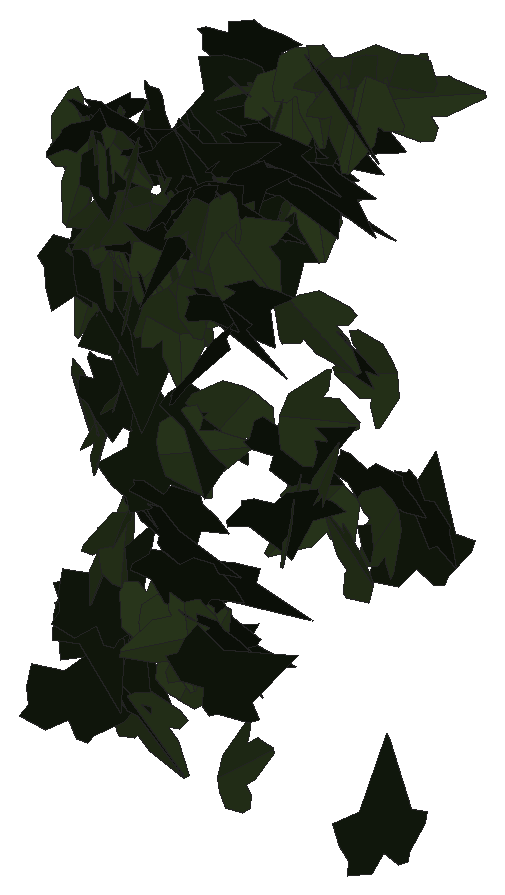
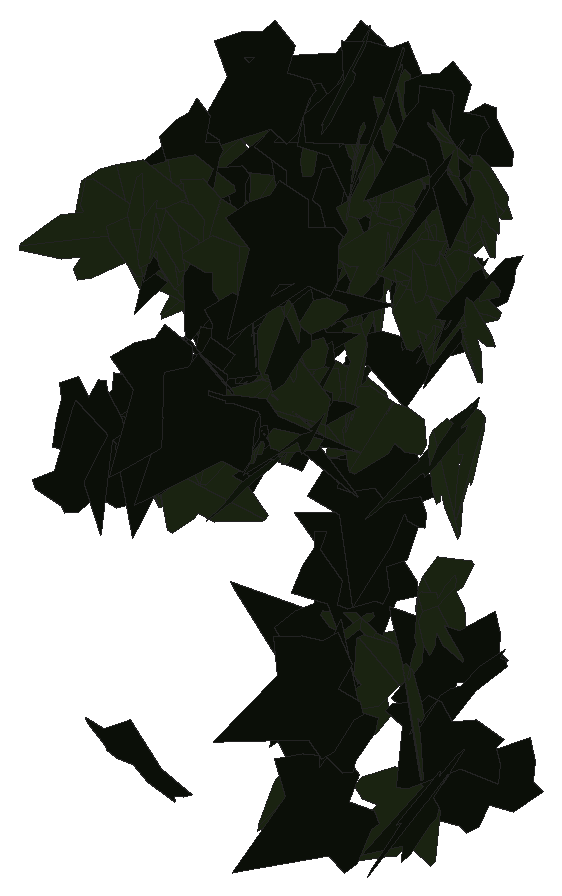
# SketchUp Ruby script. Lengths in inches.
U = 1.inch
M = Sketchup.active_model
def pt(a) = Geom::Point3d.new(a.map { |v| v * U })
def face(e, loops, mat)
  f = e.add_face(loops[0].map { |a| pt(a) })
  loops[1..].each { |l| e.add_face(l.map { |a| pt(a) }).erase! }
  f.material = f.back_material = mat if mat
  f
end
# faces: each face lists its corners as indices into pts; further lists are holes
def faces(e, pts, list, mat = nil) = list.each { |f| face(e, (f[0].is_a?(Array) ? f : [f]).map { |l| l.map { |i| pts[i] } }, mat) }
# xy, xz, yz: faces in a plane at the given z, y or x. An outline is a flat list of corners, or four numbers for a rectangle; further outlines are holes
def ring(l) = l.size == 4 ? [[l[0], l[1]], [l[2], l[1]], [l[2], l[3]], [l[0], l[3]]] : l.each_slice(2).to_a
def flat(e, list, mat, &to3) = list.each { |f| face(e, (f[0].is_a?(Array) ? f : [f]).map { |l| ring(l).map { |u, v| to3.(u, v) } }, mat) }
def xy(e, z, list, mat = nil) = flat(e, list, mat) { |x, y| [x, y, z] }
def xz(e, y, list, mat = nil) = flat(e, list, mat) { |x, z| [x, y, z] }
def yz(e, x, list, mat = nil) = flat(e, list, mat) { |y, z| [x, y, z] }
def lines(e, pts, list) = list.each { |a, b| e.add_line(pt(pts[a]), pt(pts[b])) }
# prism: a flat outline (further loops are holes) pulled along v
def prism(e, loops, v, mat = nil)
  f = face(e, loops, mat); d = Geom::Vector3d.new(v.map { |x| x * U })
  f.pushpull(f.normal.samedirection?(d) ? d.length : -d.length)
end
def box(e, o, s, mat = nil) = prism(e, [[o, [o[0] + s[0], o[1], o[2]], [o[0] + s[0], o[1] + s[1], o[2]], [o[0], o[1] + s[1], o[2]]]], [0, 0, s[2]], mat)
def at(x, y, z, deg = 0) = Geom::Transformation.translation(pt([x, y, z])) * Geom::Transformation.rotation(ORIGIN, Z_AXIS, deg.degrees)
def axes(o, x, y, z) = Geom::Transformation.new([*x, 0, *y, 0, *z, 0, *pt(o).to_a, 1])
def part(name) = M.definitions.add(name)
# library, detail: a bought-in or finely detailed component or shape, given as its bounding box
def library(name, o, s) = part(name).tap { |d| box(d.entities, o, s) }
def detail(e, o, s) = box(e.add_group.entities, o, s)
def put(e, d, t, mat = nil) = e.add_instance(d, t).tap { |i| i.material = mat if mat }
def group(e, t, mat = nil) = e.add_group.tap { |g| g.transformation = t; g.material = mat if mat }.entities
root = M.entities
M.materials.add("efeu1").color = [18, 25, 13]
M.materials.add("efeu2").color = [43, 57, 29]
c1 = part("ivyleaf_10")
p = [[0,0.5,-0.03],[-0.0625,2.02,-0.43],[-0.19,2.01,-0.46],[-0.54,1.05,-0.29],[-0.52,0.625,-0.18],[-0.83,0.76,-0.28],
  [-1.16,0.64,-0.33],[-1.15,0.33,-0.24],[-0.77,-0.39,0.02],[-0.3,-0.51,0.16],[0.04,-0.48,0.23],[-0.02,2.01,-0.4375],
  [-0.06,2.01,-0.43],[0.04,-0.49,0.23],[0.67,-0.49,0.14],[1.38,0.36,-0.2],[1.375,0.51,-0.24],[0.81,0.65,-0.19],
  [0.62,0.59,-0.15],[0.6,1.09,-0.28],[0.5,1.23,-0.31]]
faces(c1.entities,p,[[0,1,2,3,4,5,6,7,8,9,10],[11,12,0,13,14,15,16,17,18,19,20]],"efeu2")
c2 = part("ivyleaf_9")
p = [[1.54,2.16,1.25],[1.36,2.04,1.19],[-0.21,0.99,0.68],[-0.71,1.11,0.82],[-0.85,0.86,0.67],[-0.8,0.17,0.21],
  [-0.9,-0.01,0.1],[-0.67,-0.16,-0.02],[-0.08,-0.08,-0.05],[-0.03,-0.6,-0.4],[0.65,-0.88,-0.66],[0.83,-0.6,-0.49],
  [1.29,-0.42,-0.43],[1.8125,-0.07,-0.26],[1.21,0.44,0.15]]
faces(c2.entities,p,[[0,1,2,3,4,5,6,7,8,9,10,11,12,13,14]],"efeu1")
put(root,c1,axes([31.71,224.67,222.89],[0.24718,-0.43455,-0.00798],[-0.00248,0.00777,-0.49993],[0.43462,0.24719,0.00168]))
put(root,c1,axes([32.43,224.52,218.62],[0.11399,0.02563,-0.48616],[0.48525,0.0343,0.11558],[0.03927,-0.49816,-0.01706]))
put(root,c1,axes([30.8,224.67,222.25],[0.47412,-0.15396,-0.03882],[-0.03543,0.01656,-0.49847],[0.15478,0.47542,0.00479]))
put(root,c2,axes([30.73,224.47,214.24],[-0.19479,-0.11689,0.44541],[0.44193,0.08849,0.21649],[-0.12944,0.47802,0.06884]))
put(root,c2,axes([30.93,224.76,220.62],[0.25939,-0.42519,0.04395],[0.01945,-0.03961,-0.49805],[0.42701,0.26008,-0.00401]))
put(root,c1,axes([32.38,224.51,220.8125],[-0.24257,-0.36838,-0.23549],[0.15079,0.1823,-0.44049],[0.41039,-0.28472,0.02265]))
put(root,c1,axes([32.86,224.7,222.33],[-0.46609,0.17503,0.04604],[-0.1086,-0.16874,-0.45797],[-0.14478,-0.43691,0.19531]))
put(root,c2,axes([33.23,224.4,221.14],[0.34783,0.35872,-0.01827],[-0.01238,-0.01345,-0.49967],[-0.35897,0.34805,-0.00048]))
put(root,c1,axes([34.41,224.58,221.26],[-0.40164,-0.04492,-0.29439],[0.29289,0.02981,-0.40414],[0.05386,-0.49709,0.00237]))
put(root,c1,axes([31.16,224.86,216.9],[0.08879,-0.45136,0.19593],[0.05541,-0.18866,-0.45971],[0.48892,0.10335,0.01652]))
put(root,c1,axes([31.9,224.62,221.79],[-0.2401,-0.42699,-0.10015],[0.05178,0.08578,-0.48986],[0.43551,-0.2456,0.00303]))
put(root,c1,axes([32.3,225.01,215.7],[-0.07669,0.06285,0.49007],[-0.12924,-0.48122,0.04149],[0.47688,-0.12031,0.09005]))
put(root,c1,axes([32.32,224.65,220.55],[0.21033,0.45351,-0.00953],[-0.01614,-0.00301,-0.49973],[-0.45332,0.21053,0.01337]))
put(root,c1,axes([31.14,224.75,218.67],[0.1504,-0.47684,-0.00062],[-0.00017,0.00059,-0.5],[0.47684,0.1504,0.00001]))
put(root,c1,axes([30.92,224.74,220.64],[0.45441,-0.20734,-0.02286],[-0.02024,0.0107,-0.49948],[0.20761,0.45486,0.00133]))
put(root,c2,axes([32.42,224.47,222.59],[0.12712,-0.00695,0.48352],[0.4742,0.09971,-0.12323],[-0.09472,0.48991,0.03194]))
put(root,c2,axes([32.79,224.64,215.32],[0.01174,-0.00596,0.49983],[0.47668,-0.15037,-0.01299],[0.15048,0.47681,0.00215]))
put(root,c1,axes([30.81,224.58,218.9],[-0.35201,0.35299,0.03855],[-0.02671,0.0278,-0.49851],[-0.35408,-0.35302,-0.00072]))
put(root,c2,axes([32.2,224.53,217.86],[0.39157,0.21964,-0.22007],[-0.18354,-0.12237,-0.44871],[-0.25097,0.43218,-0.01521]))
put(root,c2,axes([30.82,224.8,215.8],[0.1121,-0.47584,-0.1049],[-0.01642,0.10389,-0.48881],[0.48699,0.11304,0.00766]))
put(root,c2,axes([32.41,224.93,221.93],[-0.1708,0.17047,-0.43792],[0.25145,-0.36047,-0.23839],[-0.39699,-0.30166,0.03741]))
put(root,c1,axes([32.75,224.72,222.21],[-0.05325,-0.49584,-0.03615],[0.00384,0.03595,-0.49869],[0.49714,-0.05339,-0.00003]))
put(root,c2,axes([32.83,224.33,220.01],[0.04217,0.41055,0.28226],[0.03332,0.28032,-0.41269],[-0.4971,0.05362,-0.00372]))
put(root,c2,axes([30.66,224.6,220.93],[0.1707,-0.32096,-0.34329],[-0.14958,0.30914,-0.3634],[0.44552,0.22677,0.00952]))
put(root,c2,axes([31.93,224.52,221.57],[0.3478,0.33605,-0.12691],[-0.08958,-0.08993,-0.48362],[-0.34786,0.35914,-0.00235]))
put(root,c2,axes([33.98,224.52,218.38],[0.24429,0.41669,-0.12919],[-0.08017,-0.10266,-0.48274],[-0.42883,0.25657,0.01666]))
put(root,c2,axes([32.62,224.55,222.44],[-0.07297,0.49153,-0.05541],[0.01986,-0.05305,-0.49678],[-0.49425,-0.07471,-0.01178]))
put(root,c1,axes([30.62,224.81,222.39],[0.41187,-0.21955,0.17933],[0.19745,-0.00478,-0.45934],[0.20341,0.44919,0.08276]))
put(root,c2,axes([32.49,225.07,218.91],[-0.02125,-0.43785,0.24049],[0.11804,-0.23829,-0.42342],[0.4854,0.03878,0.1135]))
put(root,c1,axes([31.375,224.89,220.61],[0.3098,-0.37447,0.11746],[0.09688,-0.07205,-0.4852],[0.38031,0.32339,0.02792]))
put(root,c2,axes([31.11,224.55,215.7],[-0.17499,-0.12318,0.45189],[0.39781,0.21554,0.21281],[-0.24723,0.43402,0.02257]))
put(root,c2,axes([31.89,224.87,217.04],[0.22565,-0.19208,0.40272],[0.34217,-0.21514,-0.29433],[0.28636,0.40843,0.03435]))
put(root,c2,axes([31.02,224.53,222.85],[0.09351,0.49073,-0.02097],[-0.00451,-0.02048,-0.49956],[-0.49116,0.09362,0.0006]))
put(root,c1,axes([32.7,224.78,222.32],[-0.39165,-0.31006,0.02171],[-0.00919,-0.02335,-0.49937],[0.31069,-0.39155,0.01259]))
put(root,c2,axes([31.94,224.51,222.8125],[0.41511,0.10171,0.2595],[0.23261,0.13003,-0.42306],[-0.15355,0.47196,0.06064]))
put(root,c1,axes([33.36,224.54,221.84],[0.14006,0.39477,0.27303],[0.04804,0.27146,-0.41714],[-0.47757,0.14308,0.03811]))
put(root,c2,axes([31.54,224.94,220.06],[-0.1901,-0.43032,-0.16937],[0.06668,0.15571,-0.47043],[0.45762,-0.20145,-0.00181]))
put(root,c1,axes([34.43,224.41,219.82],[0.01564,0.17434,0.46836],[0.00979,0.46839,-0.17468],[-0.49966,0.01464,0.01124]))
put(root,c2,axes([32.34,224.67,216.85],[0.30708,0.28473,-0.27318],[-0.21335,-0.17139,-0.41846],[-0.33194,0.37357,0.01623]))
put(root,c2,axes([32.45,224.77,223.05],[0.37247,-0.30425,-0.13674],[-0.10726,0.08485,-0.48093],[0.31585,0.3876,-0.00206]))
put(root,c2,axes([33.83,224.74,218.95],[0.4246,0.19249,-0.18074],[0.12785,0.14957,0.45965],[0.23102,-0.43655,0.07779]))
put(root,c2,axes([31.02,224.61,222.96],[0.49825,0.04137,0.00554],[0.00197,0.04302,-0.49814],[-0.04169,0.49643,0.04271]))
put(root,c1,axes([32.24,224.74,222.52],[-0.45202,0.0971,0.1904],[-0.19463,-0.00294,-0.46055],[-0.08832,-0.49047,0.04046]))
put(root,c2,axes([32.6,224.64,222.18],[0.41549,0.06904,0.26944],[0.26911,0.02263,-0.42079],[-0.0703,0.49469,-0.01836]))
put(root,c1,axes([34.58,224.84,219.2],[0.3228,-0.35463,-0.14156],[-0.09819,0.10204,-0.47953],[0.369,0.33738,-0.00376]))
put(root,c1,axes([31.09,224.92,221.34],[-0.00101,-0.49877,0.03504],[0.01326,-0.03506,-0.49859],[0.49982,-0.00008,0.0133]))
put(root,c2,axes([31.64,224.78,220.34],[0.10909,-0.26329,0.41082],[-0.17033,0.37394,0.28488],[-0.45726,-0.20211,-0.00811]))
put(root,c1,axes([30.4375,224.85,222.24],[0.31004,-0.09686,-0.38012],[0.37418,-0.07242,0.32365],[-0.11775,-0.48515,0.02758]))
put(root,c1,axes([31.17,224.92,221.54],[-0.16942,-0.4667,0.05904],[-0.02707,-0.05297,-0.49645],[0.46964,-0.17142,-0.00732]))
put(root,c2,axes([32.69,224.72,220.75],[0.49862,-0.03068,0.02099],[0.02104,0.00017,-0.49956],[0.03064,0.49906,0.00146]))
put(root,c1,axes([31.15,224.92,221.26],[0.35534,-0.08732,0.34075],[0.34693,0.00707,-0.35998],[0.05805,0.49226,0.06562]))
put(root,c1,axes([30.9,224.92,222.41],[0.10755,-0.00432,0.48828],[0.48816,-0.01082,-0.10762],[0.0115,0.49986,0.00189]))
put(root,c2,axes([31.85,224.71,223.16],[0.32303,-0.16332,-0.34493],[-0.30157,0.16771,-0.36184],[0.23389,0.44181,0.00985]))
put(root,c1,axes([32.01,224.89,215.99],[0.4313,0.08029,0.23986],[0.23655,0.03992,-0.43869],[-0.0896,0.49189,-0.00355]))
put(root,c2,axes([32.03,224.8,217.95],[-0.46424,-0.16323,0.08851],[0.08727,0.01854,0.49197],[-0.16389,0.47224,0.01128]))
put(root,c2,axes([30.95,224.75,218.99],[0.39035,-0.21757,-0.22425],[-0.10521,0.24637,-0.42218],[0.2942,0.37678,0.14656]))
put(root,c1,axes([32,224.84,221.4],[0.31732,0.37023,0.11062],[0.04997,0.10262,-0.4868],[-0.38316,0.32,0.02813]))
put(root,c2,axes([33.07,224.68,222.58],[0.19265,0.46047,-0.02912],[-0.00674,-0.02875,-0.49913],[-0.46134,0.19271,-0.00487]))
put(root,c1,axes([31.02,224.92,221.05],[-0.26169,-0.42135,-0.06312],[0.05149,0.04225,-0.49554],[0.42293,-0.26586,0.02128]))
put(root,c1,axes([31.04,225.1875,220.94],[0.10295,0.24488,-0.4236],[-0.30015,-0.31025,-0.2523],[-0.38641,0.30624,0.08312]))
put(root,c1,axes([32.37,224.76,221.79],[-0.17324,0.39852,-0.24732],[-0.09138,0.22992,0.43449],[0.46004,0.19575,-0.00683]))
put(root,c1,axes([33.8,225.15,218.31],[0.30782,-0.32876,0.21718],[0.15483,-0.1525,-0.4503],[0.36232,0.34447,0.00791]))
put(root,c1,axes([31.91,224.9,221.05],[-0.39361,0.28512,0.11738],[-0.13942,0.00519,-0.48014],[-0.27501,-0.41071,0.07541]))
put(root,c2,axes([30.99,224.69,222.38],[0.23386,-0.05565,-0.43842],[-0.28822,0.35681,-0.19904],[0.33502,0.34582,0.13481]))
put(root,c1,axes([32.55,224.65,220.92],[-0.04219,0.26524,0.42174],[-0.09425,0.41136,-0.26814],[-0.48922,-0.10212,0.01529]))
put(root,c1,axes([31.8,224.84,221.11],[0.10607,0.43059,0.23096],[-0.00839,0.23791,-0.43969],[-0.48855,0.0894,0.0577]))
put(root,c2,axes([32.61,224.79,222.13],[0.2866,0.40969,-0.00434],[-0.02967,0.01547,-0.49888],[-0.40864,0.28621,0.03318]))
put(root,c1,axes([31.23,224.82,216.41],[-0.04548,0.37707,-0.32519],[-0.0379,0.32297,0.37981],[0.49648,0.0592,-0.0008]))
put(root,c1,axes([32.91,225.14,219.15],[0.35815,0.2033,-0.28355],[-0.30759,-0.00782,-0.39412],[-0.16468,0.45674,0.11946]))
put(root,c2,axes([32.44,224.95,215.92],[0.48132,0.08076,-0.10867],[-0.10919,-0.00577,-0.4879],[-0.08006,0.4934,0.01208]))
put(root,c2,axes([30.71,225.13,215.5],[-0.16003,-0.21578,-0.4217],[0.29044,0.30693,-0.26727],[0.37421,-0.3305,0.02711]))
put(root,c1,axes([31.35,225.08,214.26],[-0.42297,0.03054,-0.26489],[0.26475,-0.01103,-0.42401],[-0.03174,-0.49894,-0.00684]))
put(root,c2,axes([34.45,224.98,220.81],[0.47191,0.02614,-0.16314],[-0.16364,0.00579,-0.47243],[-0.02281,0.49928,0.01401]))
put(root,c1,axes([34.97,224.96,217.59],[-0.12025,0.12192,-0.46976],[-0.37205,0.28761,0.16989],[0.31164,0.39041,0.02155]))
put(root,c1,axes([31.03,224.99,221.29],[0.13325,0.45104,0.16973],[0.02263,0.17005,-0.46965],[-0.48139,0.13284,0.0249]))
put(root,c2,axes([30.93,225.22,214.52],[0.39855,-0.30185,0.00659],[0.00533,-0.00387,-0.49996],[0.30187,0.39859,0.00013]))
put(root,c1,axes([31.68,224.93,215.68],[0.2197,0.3416,-0.29161],[0.09439,0.28226,0.40177],[0.43911,-0.23159,0.05954]))
put(root,c1,axes([32.95,224.94,213.98],[-0.00932,0.05484,0.4969],[-0.17921,0.46359,-0.05452],[-0.46669,-0.17911,0.01102]))
put(root,c1,axes([32.06,225.14,214.93],[0.1791,0.32659,-0.33356],[0.17331,0.28522,0.37231],[0.43346,-0.24898,-0.01104]))
put(root,c1,axes([35.02,225.33,220.29],[0.19775,-0.08372,-0.45154],[-0.40267,0.20476,-0.21431],[0.2208,0.4484,0.01356]))
put(root,c2,axes([33.05,225.21,223.01],[0.48256,0.10851,0.07325],[0.06797,0.03145,-0.49436],[-0.11189,0.48707,0.0156]))
put(root,c1,axes([31.12,225.33,215.92],[0.27496,-0.32756,-0.25904],[-0.12417,0.23199,-0.42516],[0.39872,0.29813,0.04624]))
put(root,c2,axes([35.11,225.27,213.53],[-0.48235,0.13158,0.00531],[0.00298,-0.00926,0.49991],[0.13166,0.48229,0.00815]))
put(root,c1,axes([34.97,225.5,218.08],[0.37027,-0.23776,-0.23742],[-0.18467,0.15114,-0.43938],[0.2807,0.41307,0.02411]))
put(root,c1,axes([33.8,225.8,217.83],[0.21674,0.24531,-0.37795],[-0.2821,-0.25316,-0.32608],[-0.35135,0.35459,0.02867]))
put(root,c2,axes([30.61,225.51,214.99],[0.28574,-0.30865,-0.27036],[-0.13424,0.241,-0.41701],[0.38773,0.3109,0.05485]))
put(root,c2,axes([34.49,225.74,218.49],[0.3854,0.16469,-0.27267],[-0.24584,-0.11837,-0.41898],[-0.20256,0.45702,-0.01027]))
put(root,c2,axes([31.71,226.08,215.24],[0.47058,-0.14633,0.08453],[-0.07245,0.05127,0.49206],[-0.15267,-0.47535,0.02705]))
put(root,c2,axes([35.3,225.84,218.31],[0.26373,0.05331,-0.42143],[-0.41504,-0.07333,-0.26901],[-0.09049,0.49171,0.00557]))
put(root,c1,axes([30.96,225.96,219.75],[0.39068,0.19693,0.24206],[0.21474,0.11174,-0.43749],[-0.2264,0.4458,0.00273]))
put(root,c2,axes([35.1,225.95,217.3],[-0.34944,-0.16724,0.31611],[0.31489,0.06561,0.38281],[-0.16952,0.46661,0.05947]))
put(root,c2,axes([31.75,225.94,215.94],[0.44807,0.07979,0.20704],[0.20086,0.05235,-0.45488],[-0.09427,0.49081,0.01486]))
put(root,c1,axes([31.39,225.92,220.26],[-0.03151,0.1341,0.48065],[-0.32989,0.35575,-0.12088],[-0.37441,-0.32474,0.06606]))
put(root,c2,axes([33.23,226.19,222.15],[0.46885,0.15327,-0.08175],[-0.08507,-0.00257,-0.4927],[-0.15146,0.47592,0.02367]))
put(root,c2,axes([31.42,226.15,214.7],[0.35978,0.24981,0.24116],[0.19192,0.14633,-0.4379],[-0.28936,0.40766,0.00941]))
put(root,c2,axes([32.76,226.48,221.79],[0.3821,0.30134,-0.11484],[-0.09322,-0.06724,-0.48661],[-0.30872,0.39328,0.0048]))
put(root,c2,axes([32.77,226.99,222.98],[0.46085,-0.08597,-0.17385],[-0.17223,0.02467,-0.46875],[0.08917,0.49194,-0.00687]))
put(root,c2,axes([31.08,227.67,221.75],[-0.2729,-0.25422,0.33301],[-0.24562,-0.22488,-0.37296],[0.3394,-0.36715,-0.00214]))
put(root,c2,axes([31.08,227.625,221.18],[-0.16833,-0.46964,0.03327],[0.01692,-0.04134,-0.498],[0.47051,-0.16653,0.02981]))
put(root,c1,axes([32.06,227.55,222.66],[0.45434,0.01428,0.20825],[0.20743,0.0248,-0.45427],[-0.02331,0.49918,0.01661]))
put(root,c2,axes([31.46,227.58,221.61],[0.1185,0.2382,-0.42334],[-0.22881,-0.35701,-0.26493],[-0.42849,0.25652,0.0244]))
put(root,c1,axes([32.7,227.62,222.81],[-0.26226,-0.42176,0.05778],[-0.02405,-0.05308,-0.49659],[0.42502,-0.26326,0.00755]))
put(root,c1,axes([30.94,227.73,221.69],[-0.12512,-0.45643,0.16131],[-0.00509,-0.16536,-0.47184],[0.48406,-0.11972,0.03674]))
put(root,c1,axes([32.66,227.72,222.48],[-0.08067,-0.48084,0.11083],[0.11591,-0.12762,-0.46934],[0.47964,-0.05003,0.13206]))
put(root,c2,axes([30.89,227.83,220.47],[-0.12219,-0.48376,-0.03233],[0.01438,0.02971,-0.49891],[0.48463,-0.12285,0.00665]))
put(root,c1,axes([31.71,227.625,222.1875],[0.46357,0.17635,0.06325],[0.05445,0.03469,-0.49581],[-0.17926,0.46658,0.01296]))
put(root,c1,axes([32.79,227.68,222.44],[0.48982,0.0998,-0.01071],[-0.00862,-0.01135,-0.4998],[-0.10001,0.48981,-0.0094]))
put(root,c1,axes([31.6,227.53,221.93],[0.17489,-0.39912,-0.24519],[-0.08078,0.2321,-0.43543],[0.4614,0.19192,0.0167]))
put(root,c2,axes([31.15,227.8,220.55],[-0.49971,0.01695,0.00216],[-0.00185,0.00944,-0.49991],[-0.01699,-0.49962,-0.00937]))
put(root,c2,axes([30.58,227.64,220.91],[0.44151,-0.21535,-0.09325],[-0.07678,0.05519,-0.49098],[0.22175,0.44786,0.01566]))
put(root,c2,axes([30.92,227.48,222.76],[0.4394,0.23842,-0.00907],[-0.00825,-0.00382,-0.49992],[-0.23845,0.43948,0.00058]))
put(root,c1,axes([31.03,227.77,221.73],[-0.42021,0.20119,-0.1815],[0.1449,-0.11616,-0.46423],[-0.22896,-0.44275,0.03932]))
put(root,c1,axes([30.73,227.67,220.9375],[0.15099,0.46261,0.11487],[0.00964,0.1175,-0.4859],[-0.47656,0.14894,0.02656]))
put(root,c1,axes([31.43,227.74,220.91],[-0.44821,0.15615,0.15723],[-0.15331,0.03763,-0.47443],[-0.16,-0.4735,0.01415]))
put(root,c2,axes([30.8,227.82,221.75],[0.46847,-0.16541,0.05639],[0.0641,0.01255,-0.49572],[0.16258,0.47168,0.03296]))
put(root,c2,axes([31.08,228.16,219.84],[0.06045,-0.47944,0.12837],[0.0913,-0.11637,-0.47762],[0.48786,0.08118,0.07348]))
put(root,c2,axes([31.58,227.91,220.7],[0.43867,-0.12779,0.20308],[0.21126,0.00509,-0.45315],[0.11374,0.48337,0.05846]))
put(root,c1,axes([33.07,228.07,222.82],[-0.38345,-0.28723,0.14307],[-0.12343,-0.07375,-0.47888],[0.2962,-0.40257,-0.01435]))
put(root,c1,axes([30.52,227.97,220.75],[-0.06681,-0.02077,0.49508],[0.41912,0.26413,0.06764],[-0.26434,0.42403,-0.01788]))
put(root,c2,axes([31.27,228.25,220.62],[-0.37807,0.08682,0.31547],[-0.32411,-0.03324,-0.37927],[-0.04488,-0.49128,0.08141]))
put(root,c2,axes([31.78,228.26,221.21],[-0.47009,0.1702,-0.0071],[0.00864,0.00303,-0.49992],[-0.17013,-0.47013,-0.00579]))
put(root,c1,axes([31.53,228.28,220.5],[0.43815,0.20044,0.13362],[0.12321,0.05185,-0.4818],[-0.207,0.45512,-0.00396]))
put(root,c2,axes([31.4,228.18,220.91],[0.47649,0.12928,-0.07902],[-0.07951,-0.00865,-0.49356],[-0.12898,0.48292,0.01231]))
put(root,c1,axes([33.11,228.19,222.27],[0.00089,-0.01108,0.49988],[0.22439,0.44672,0.00951],[-0.44682,0.22432,0.00577]))
put(root,c2,axes([31.24,228.57,220.9],[0.38985,0.30002,0.08946],[0.05417,0.07607,-0.4912],[-0.30835,0.39269,0.02681]))
put(root,c2,axes([31.7,228.59,221.11],[0.27384,0.38424,0.16544],[0.08948,0.13935,-0.47178],[-0.40866,0.28799,0.00756]))
